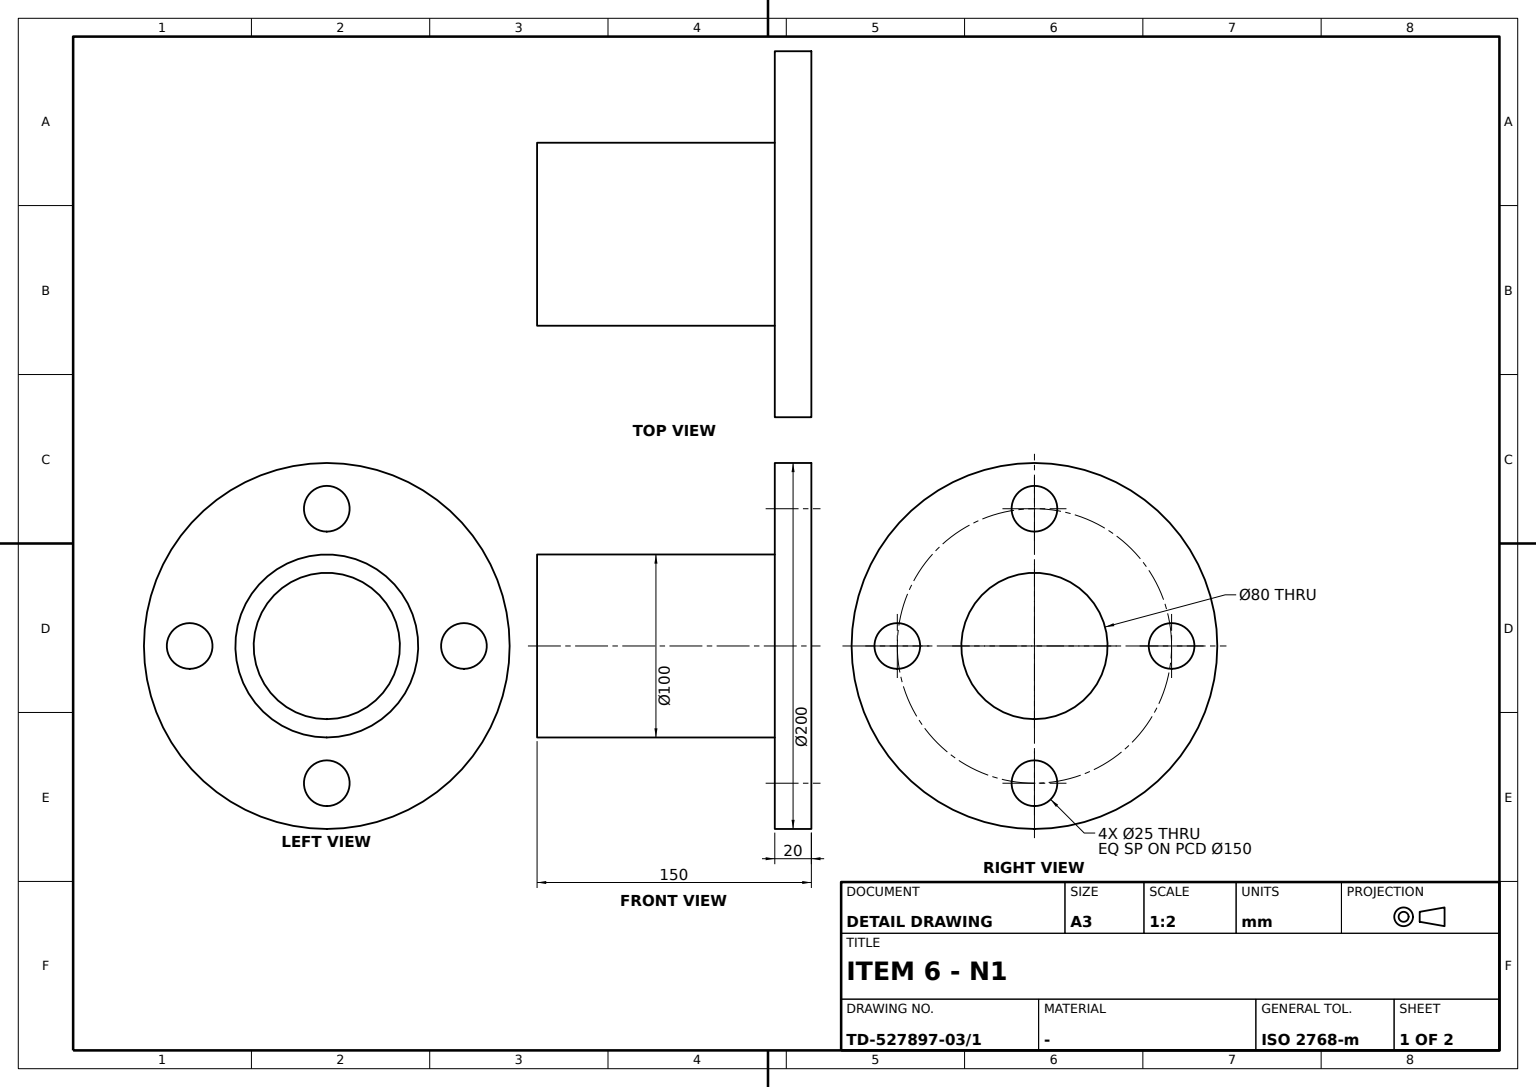
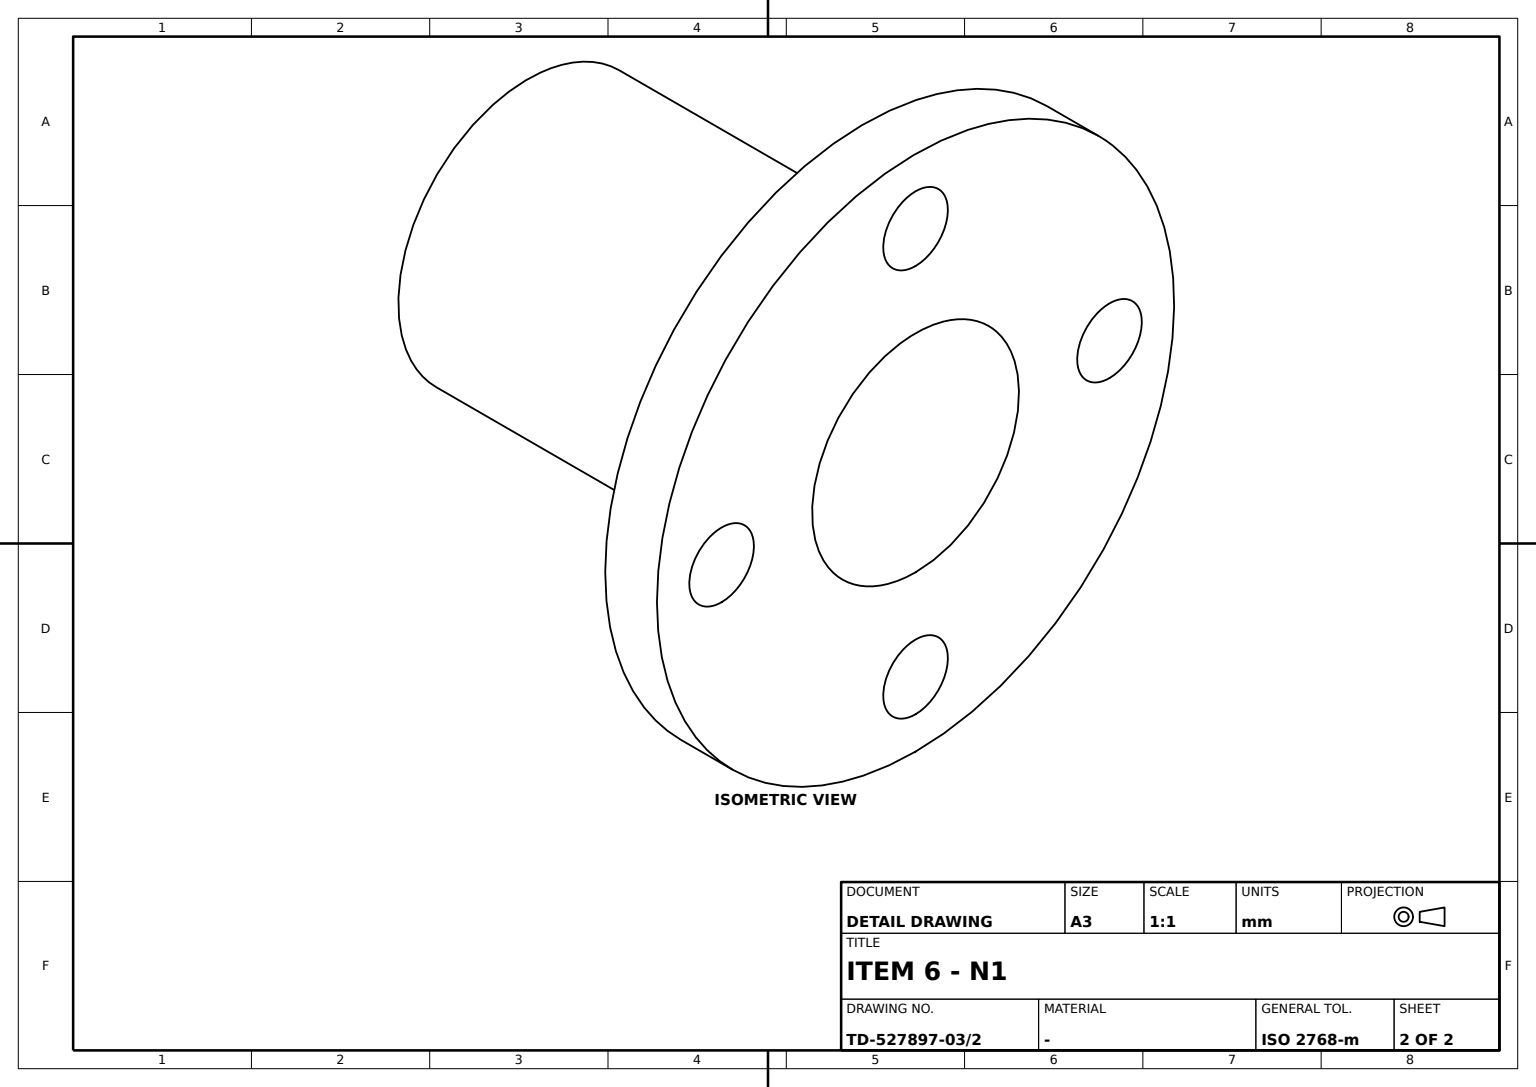
ISO-10303-21;
HEADER;
FILE_DESCRIPTION((''),'2;1');
FILE_NAME('','',(''),(''),'','','');
FILE_SCHEMA(('AUTOMOTIVE_DESIGN'));
ENDSEC;
DATA;
#1=APPLICATION_CONTEXT('');
#2=PRODUCT_CONTEXT('',#1,'mechanical');
#3=PRODUCT('','','',(#2));
#4=PRODUCT_DEFINITION_FORMATION('','',#3);
#5=PRODUCT_DEFINITION_CONTEXT('',#1,'design');
#6=PRODUCT_DEFINITION('','',#4,#5);
#7=PRODUCT_DEFINITION_SHAPE('','',#6);
#8=(LENGTH_UNIT()NAMED_UNIT(*)SI_UNIT(.MILLI.,.METRE.));
#9=(NAMED_UNIT(*)PLANE_ANGLE_UNIT()SI_UNIT($,.RADIAN.));
#10=(NAMED_UNIT(*)SI_UNIT($,.STERADIAN.)SOLID_ANGLE_UNIT());
#11=UNCERTAINTY_MEASURE_WITH_UNIT(LENGTH_MEASURE(0.005),#8,'distance_accuracy_value','');
#12=(GEOMETRIC_REPRESENTATION_CONTEXT(3)GLOBAL_UNCERTAINTY_ASSIGNED_CONTEXT((#11))GLOBAL_UNIT_ASSIGNED_CONTEXT((#8,#9,#10))REPRESENTATION_CONTEXT('',''));
#13=CARTESIAN_POINT('',(-1200.,1250.,2500.));
#14=VERTEX_POINT('',#13);
#15=CARTESIAN_POINT('',(-1250.,1250.,2500.));
#16=DIRECTION('',(0.,0.,1.));
#17=DIRECTION('',(1.,0.,0.));
#18=AXIS2_PLACEMENT_3D('',#15,#16,#17);
#19=CIRCLE('',#18,50.);
#20=EDGE_CURVE('',#14,#14,#19,.T.);
#21=ORIENTED_EDGE('',*,*,#20,.F.);
#22=EDGE_LOOP('',(#21));
#23=FACE_BOUND('',#22,.T.);
#24=CARTESIAN_POINT('',(-1210.,1250.,2500.));
#25=VERTEX_POINT('',#24);
#26=CIRCLE('',#18,40.);
#27=EDGE_CURVE('',#25,#25,#26,.T.);
#28=ORIENTED_EDGE('',*,*,#27,.T.);
#29=EDGE_LOOP('',(#28));
#30=FACE_BOUND('',#29,.T.);
#31=CARTESIAN_POINT('',(0.,0.,2500.));
#32=AXIS2_PLACEMENT_3D('',#31,#16,#17);
#33=PLANE('',#32);
#34=ADVANCED_FACE('',(#23,#30),#33,.F.);
#35=CARTESIAN_POINT('',(-1150.,1250.,2650.));
#36=VERTEX_POINT('',#35);
#37=CARTESIAN_POINT('',(-1250.,1250.,2650.));
#38=AXIS2_PLACEMENT_3D('',#37,#16,#17);
#39=CIRCLE('',#38,100.);
#40=EDGE_CURVE('',#36,#36,#39,.T.);
#41=ORIENTED_EDGE('',*,*,#40,.T.);
#42=EDGE_LOOP('',(#41));
#43=FACE_BOUND('',#42,.T.);
#44=CARTESIAN_POINT('',(-1237.5,1325.,2650.));
#45=VERTEX_POINT('',#44);
#46=CARTESIAN_POINT('',(-1250.,1325.,2650.));
#47=AXIS2_PLACEMENT_3D('',#46,#16,#17);
#48=CIRCLE('',#47,12.5);
#49=EDGE_CURVE('',#45,#45,#48,.T.);
#50=ORIENTED_EDGE('',*,*,#49,.F.);
#51=EDGE_LOOP('',(#50));
#52=FACE_BOUND('',#51,.T.);
#53=CARTESIAN_POINT('',(-1210.,1250.,2650.));
#54=VERTEX_POINT('',#53);
#55=CIRCLE('',#38,40.);
#56=EDGE_CURVE('',#54,#54,#55,.T.);
#57=ORIENTED_EDGE('',*,*,#56,.F.);
#58=EDGE_LOOP('',(#57));
#59=FACE_BOUND('',#58,.T.);
#60=CARTESIAN_POINT('',(-1312.5,1250.,2650.));
#61=VERTEX_POINT('',#60);
#62=CARTESIAN_POINT('',(-1325.,1250.,2650.));
#63=AXIS2_PLACEMENT_3D('',#62,#16,#17);
#64=CIRCLE('',#63,12.5);
#65=EDGE_CURVE('',#61,#61,#64,.T.);
#66=ORIENTED_EDGE('',*,*,#65,.F.);
#67=EDGE_LOOP('',(#66));
#68=FACE_BOUND('',#67,.T.);
#69=CARTESIAN_POINT('',(-1237.5,1175.,2650.));
#70=VERTEX_POINT('',#69);
#71=CARTESIAN_POINT('',(-1250.,1175.,2650.));
#72=AXIS2_PLACEMENT_3D('',#71,#16,#17);
#73=CIRCLE('',#72,12.5);
#74=EDGE_CURVE('',#70,#70,#73,.T.);
#75=ORIENTED_EDGE('',*,*,#74,.F.);
#76=EDGE_LOOP('',(#75));
#77=FACE_BOUND('',#76,.T.);
#78=CARTESIAN_POINT('',(-1162.5,1250.,2650.));
#79=VERTEX_POINT('',#78);
#80=CARTESIAN_POINT('',(-1175.,1250.,2650.));
#81=AXIS2_PLACEMENT_3D('',#80,#16,#17);
#82=CIRCLE('',#81,12.5);
#83=EDGE_CURVE('',#79,#79,#82,.T.);
#84=ORIENTED_EDGE('',*,*,#83,.F.);
#85=EDGE_LOOP('',(#84));
#86=FACE_BOUND('',#85,.T.);
#87=CARTESIAN_POINT('',(0.,0.,2650.));
#88=AXIS2_PLACEMENT_3D('',#87,#16,#17);
#89=PLANE('',#88);
#90=ADVANCED_FACE('',(#43,#52,#59,#68,#77,#86),#89,.T.);
#91=CARTESIAN_POINT('',(-1200.,1250.,2630.));
#92=VERTEX_POINT('',#91);
#93=CARTESIAN_POINT('',(-1250.,1250.,2630.));
#94=AXIS2_PLACEMENT_3D('',#93,#16,#17);
#95=CIRCLE('',#94,50.);
#96=EDGE_CURVE('',#92,#92,#95,.T.);
#97=ORIENTED_EDGE('',*,*,#96,.F.);
#98=EDGE_LOOP('',(#97));
#99=FACE_BOUND('',#98,.T.);
#100=ORIENTED_EDGE('',*,*,#20,.T.);
#101=EDGE_LOOP('',(#100));
#102=FACE_BOUND('',#101,.T.);
#103=CARTESIAN_POINT('',(-1250.,1250.,2575.));
#104=AXIS2_PLACEMENT_3D('',#103,#16,#17);
#105=CYLINDRICAL_SURFACE('',#104,50.);
#106=ADVANCED_FACE('',(#99,#102),#105,.T.);
#107=ORIENTED_EDGE('',*,*,#49,.T.);
#108=EDGE_LOOP('',(#107));
#109=FACE_BOUND('',#108,.T.);
#110=CARTESIAN_POINT('',(-1237.5,1325.,2630.));
#111=VERTEX_POINT('',#110);
#112=CARTESIAN_POINT('',(-1250.,1325.,2630.));
#113=AXIS2_PLACEMENT_3D('',#112,#16,#17);
#114=CIRCLE('',#113,12.5);
#115=EDGE_CURVE('',#111,#111,#114,.T.);
#116=ORIENTED_EDGE('',*,*,#115,.F.);
#117=EDGE_LOOP('',(#116));
#118=FACE_BOUND('',#117,.T.);
#119=CARTESIAN_POINT('',(-1250.,1325.,2640.));
#120=AXIS2_PLACEMENT_3D('',#119,#16,#17);
#121=CYLINDRICAL_SURFACE('',#120,12.5);
#122=ADVANCED_FACE('',(#109,#118),#121,.F.);
#123=ORIENTED_EDGE('',*,*,#65,.T.);
#124=EDGE_LOOP('',(#123));
#125=FACE_BOUND('',#124,.T.);
#126=CARTESIAN_POINT('',(-1312.5,1250.,2630.));
#127=VERTEX_POINT('',#126);
#128=CARTESIAN_POINT('',(-1325.,1250.,2630.));
#129=AXIS2_PLACEMENT_3D('',#128,#16,#17);
#130=CIRCLE('',#129,12.5);
#131=EDGE_CURVE('',#127,#127,#130,.T.);
#132=ORIENTED_EDGE('',*,*,#131,.F.);
#133=EDGE_LOOP('',(#132));
#134=FACE_BOUND('',#133,.T.);
#135=CARTESIAN_POINT('',(-1325.,1250.,2640.));
#136=AXIS2_PLACEMENT_3D('',#135,#16,#17);
#137=CYLINDRICAL_SURFACE('',#136,12.5);
#138=ADVANCED_FACE('',(#125,#134),#137,.F.);
#139=ORIENTED_EDGE('',*,*,#40,.F.);
#140=EDGE_LOOP('',(#139));
#141=FACE_BOUND('',#140,.T.);
#142=CARTESIAN_POINT('',(-1150.,1250.,2630.));
#143=VERTEX_POINT('',#142);
#144=CIRCLE('',#94,100.);
#145=EDGE_CURVE('',#143,#143,#144,.T.);
#146=ORIENTED_EDGE('',*,*,#145,.T.);
#147=EDGE_LOOP('',(#146));
#148=FACE_BOUND('',#147,.T.);
#149=CARTESIAN_POINT('',(-1250.,1250.,2640.));
#150=AXIS2_PLACEMENT_3D('',#149,#16,#17);
#151=CYLINDRICAL_SURFACE('',#150,100.);
#152=ADVANCED_FACE('',(#141,#148),#151,.T.);
#153=ORIENTED_EDGE('',*,*,#56,.T.);
#154=EDGE_LOOP('',(#153));
#155=FACE_BOUND('',#154,.T.);
#156=ORIENTED_EDGE('',*,*,#27,.F.);
#157=EDGE_LOOP('',(#156));
#158=FACE_BOUND('',#157,.T.);
#159=CYLINDRICAL_SURFACE('',#150,40.);
#160=ADVANCED_FACE('',(#155,#158),#159,.F.);
#161=ORIENTED_EDGE('',*,*,#115,.T.);
#162=EDGE_LOOP('',(#161));
#163=FACE_BOUND('',#162,.T.);
#164=ORIENTED_EDGE('',*,*,#145,.F.);
#165=EDGE_LOOP('',(#164));
#166=FACE_BOUND('',#165,.T.);
#167=CARTESIAN_POINT('',(-1237.5,1175.,2630.));
#168=VERTEX_POINT('',#167);
#169=CARTESIAN_POINT('',(-1250.,1175.,2630.));
#170=AXIS2_PLACEMENT_3D('',#169,#16,#17);
#171=CIRCLE('',#170,12.5);
#172=EDGE_CURVE('',#168,#168,#171,.T.);
#173=ORIENTED_EDGE('',*,*,#172,.T.);
#174=EDGE_LOOP('',(#173));
#175=FACE_BOUND('',#174,.T.);
#176=CARTESIAN_POINT('',(-1162.5,1250.,2630.));
#177=VERTEX_POINT('',#176);
#178=CARTESIAN_POINT('',(-1175.,1250.,2630.));
#179=AXIS2_PLACEMENT_3D('',#178,#16,#17);
#180=CIRCLE('',#179,12.5);
#181=EDGE_CURVE('',#177,#177,#180,.T.);
#182=ORIENTED_EDGE('',*,*,#181,.T.);
#183=EDGE_LOOP('',(#182));
#184=FACE_BOUND('',#183,.T.);
#185=ORIENTED_EDGE('',*,*,#131,.T.);
#186=EDGE_LOOP('',(#185));
#187=FACE_BOUND('',#186,.T.);
#188=ORIENTED_EDGE('',*,*,#96,.T.);
#189=EDGE_LOOP('',(#188));
#190=FACE_BOUND('',#189,.T.);
#191=CARTESIAN_POINT('',(0.,0.,2630.));
#192=AXIS2_PLACEMENT_3D('',#191,#16,#17);
#193=PLANE('',#192);
#194=ADVANCED_FACE('',(#163,#166,#175,#184,#187,#190),#193,.F.);
#195=ORIENTED_EDGE('',*,*,#181,.F.);
#196=EDGE_LOOP('',(#195));
#197=FACE_BOUND('',#196,.T.);
#198=ORIENTED_EDGE('',*,*,#83,.T.);
#199=EDGE_LOOP('',(#198));
#200=FACE_BOUND('',#199,.T.);
#201=CARTESIAN_POINT('',(-1175.,1250.,2640.));
#202=AXIS2_PLACEMENT_3D('',#201,#16,#17);
#203=CYLINDRICAL_SURFACE('',#202,12.5);
#204=ADVANCED_FACE('',(#197,#200),#203,.F.);
#205=ORIENTED_EDGE('',*,*,#74,.T.);
#206=EDGE_LOOP('',(#205));
#207=FACE_BOUND('',#206,.T.);
#208=ORIENTED_EDGE('',*,*,#172,.F.);
#209=EDGE_LOOP('',(#208));
#210=FACE_BOUND('',#209,.T.);
#211=CARTESIAN_POINT('',(-1250.,1175.,2640.));
#212=AXIS2_PLACEMENT_3D('',#211,#16,#17);
#213=CYLINDRICAL_SURFACE('',#212,12.5);
#214=ADVANCED_FACE('',(#207,#210),#213,.F.);
#215=CLOSED_SHELL('',(#34,#90,#106,#122,#138,#152,#160,#194,#204,#214));
#216=MANIFOLD_SOLID_BREP('',#215);
#217=ADVANCED_BREP_SHAPE_REPRESENTATION('',(#216),#12);
#218=SHAPE_DEFINITION_REPRESENTATION(#7,#217);
ENDSEC;
END-ISO-10303-21;
